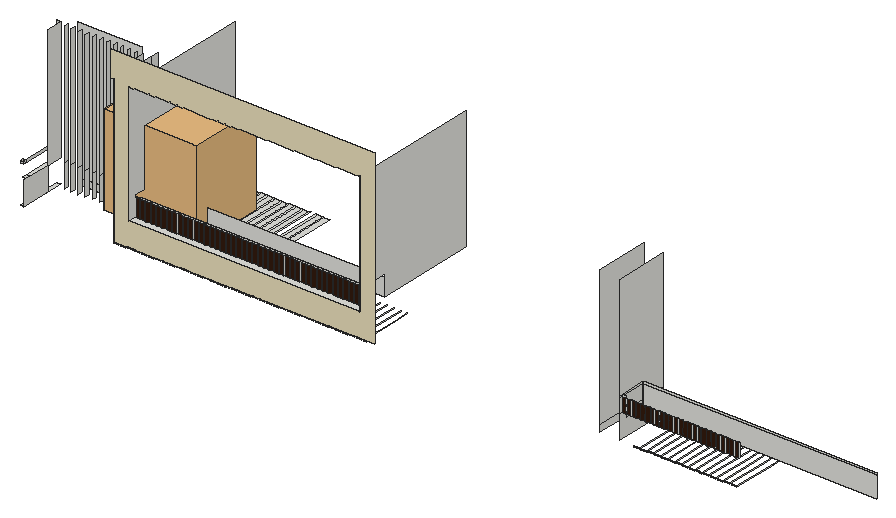
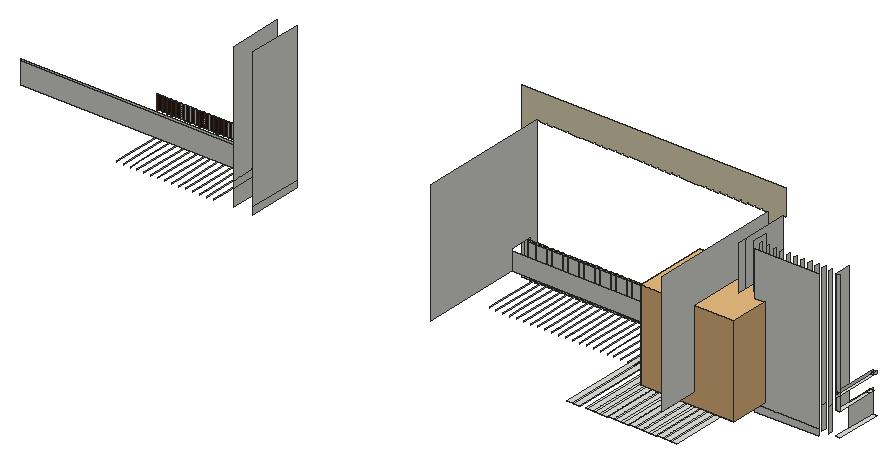
# SketchUp Ruby script. Lengths in inches.
U = 1.inch
M = Sketchup.active_model
def pt(a) = Geom::Point3d.new(a.map { |v| v * U })
def face(e, loops, mat)
  f = e.add_face(loops[0].map { |a| pt(a) })
  loops[1..].each { |l| e.add_face(l.map { |a| pt(a) }).erase! }
  f.material = f.back_material = mat if mat
  f
end
# faces: each face lists its corners as indices into pts; further lists are holes
def faces(e, pts, list, mat = nil) = list.each { |f| face(e, (f[0].is_a?(Array) ? f : [f]).map { |l| l.map { |i| pts[i] } }, mat) }
# xy, xz, yz: faces in a plane at the given z, y or x. An outline is a flat list of corners, or four numbers for a rectangle; further outlines are holes
def ring(l) = l.size == 4 ? [[l[0], l[1]], [l[2], l[1]], [l[2], l[3]], [l[0], l[3]]] : l.each_slice(2).to_a
def flat(e, list, mat, &to3) = list.each { |f| face(e, (f[0].is_a?(Array) ? f : [f]).map { |l| ring(l).map { |u, v| to3.(u, v) } }, mat) }
def xy(e, z, list, mat = nil) = flat(e, list, mat) { |x, y| [x, y, z] }
def xz(e, y, list, mat = nil) = flat(e, list, mat) { |x, z| [x, y, z] }
def yz(e, x, list, mat = nil) = flat(e, list, mat) { |y, z| [x, y, z] }
def lines(e, pts, list) = list.each { |a, b| e.add_line(pt(pts[a]), pt(pts[b])) }
# prism: a flat outline (further loops are holes) pulled along v
def prism(e, loops, v, mat = nil)
  f = face(e, loops, mat); d = Geom::Vector3d.new(v.map { |x| x * U })
  f.pushpull(f.normal.samedirection?(d) ? d.length : -d.length)
end
def box(e, o, s, mat = nil) = prism(e, [[o, [o[0] + s[0], o[1], o[2]], [o[0] + s[0], o[1] + s[1], o[2]], [o[0], o[1] + s[1], o[2]]]], [0, 0, s[2]], mat)
def at(x, y, z, deg = 0) = Geom::Transformation.translation(pt([x, y, z])) * Geom::Transformation.rotation(ORIGIN, Z_AXIS, deg.degrees)
def axes(o, x, y, z) = Geom::Transformation.new([*x, 0, *y, 0, *z, 0, *pt(o).to_a, 1])
def part(name) = M.definitions.add(name)
# library, detail: a bought-in or finely detailed component or shape, given as its bounding box
def library(name, o, s) = part(name).tap { |d| box(d.entities, o, s) }
def detail(e, o, s) = box(e.add_group.entities, o, s)
def put(e, d, t, mat = nil) = e.add_instance(d, t).tap { |i| i.material = mat if mat }
def group(e, t, mat = nil) = e.add_group.tap { |g| g.transformation = t; g.material = mat if mat }.entities
root = M.entities
M.materials.add("[Color D01]").color = [237, 225, 189]
M.materials.add("[Wood Veneer 01]").color = [51, 28, 15]
c1 = library("Round Planter with Plant",[-35.48,-39.77,0],[80.62,63.55,77.875])
xy(root,254.6875,[[1049,246.64,1052.37,286.21],[1130.14,246.64,1134.52,361.27],[1134.52,246.64,1136.14,361.27],[1136.14,246.64,1140.52,361.27],[1140.52,246.64,1142.14,361.27],
  [1142.14,246.64,1146.52,361.27],[1146.52,246.64,1148.14,361.27],[1148.14,246.64,1152.52,361.27],[1152.52,246.64,1154.14,361.27],[1154.14,246.64,1158.52,361.27],
  [1158.52,246.64,1160.14,361.27],[1160.14,246.64,1164.52,361.27],[1164.52,246.64,1166.14,361.27],[1166.14,246.64,1170.52,361.27],[1170.52,246.64,1172.14,361.27],
  [1172.14,246.64,1176.52,361.27],[1176.52,246.64,1178.14,361.27],[1178.14,246.64,1182.52,361.27],[1182.52,246.64,1184.14,361.27],[1184.14,246.64,1188.52,361.27],
  [1188.52,246.64,1190.14,361.27],[1190.14,246.64,1194.52,361.27],[1194.52,246.64,1196.14,361.27],[1196.14,246.64,1200.52,361.27],[1200.52,246.64,1202.14,361.27],
  [1202.14,246.64,1206.52,361.27],[1206.52,246.64,1208.14,361.27],[1212.52,246.64,1214.14,361.27],[1214.14,246.64,1218.52,361.27],[1218.52,246.64,1220.14,361.27],
  [1220.14,246.64,1224.52,361.27]])
xy(root,275.125,[[1142.89,246.64,1342.64,246.64,1342.64,255.84,1146.57,255.84,1146.57,253.84,1142.89,253.84],[1049,249.27,1052.37,253.58],[1049,253.58,1052.37,286.21],[1142.89,253.84,1146.57,255.47]])
xy(root,287.25,[[1049,246.64,1051.625,249.27],[1049,249.27,1051.625,286.21]])
xz(root,246.64,[[1049,287.25,1051.625,289.1875]])
xz(root,246.64,[[[1130.14,254.6875,1355.5625,254.6875,1355.5625,403.1875,1127.51,403.1875,1127.51,380.6875,1130.14,380.6875],[1142.89,275.125,1142.89,379.5625,1147.3,379.5625,1147.3,380.6875,1148.89,380.6875,1148.89,379.5625,1153.3,379.5625,1153.3,380.6875,1154.89,380.6875,1154.89,379.5625,1159.3,379.5625,1159.3,380.6875,1160.89,380.6875,1160.89,379.5625,1165.3,379.5625,1165.3,380.6875,1166.89,380.6875,1166.89,379.5625,1171.3,379.5625,1171.3,380.6875,1172.89,380.6875,1172.89,379.5625,1177.3,379.5625,1177.3,380.6875,1178.89,380.6875,1178.89,379.5625,1183.3,379.5625,1183.3,380.6875,1184.89,380.6875,1184.89,379.5625,1189.3,379.5625,1189.3,380.6875,1190.89,380.6875,1190.89,379.5625,1195.3,379.5625,1195.3,380.6875,1196.89,380.6875,1196.89,379.5625,1201.3,379.5625,1201.3,380.6875,1202.89,380.6875,1202.89,379.5625,1207.3,379.5625,1207.3,380.6875,1208.89,380.6875,1208.89,379.5625,1213.3,379.5625,1213.3,380.6875,1214.89,380.6875,1214.89,379.5625,1219.3,379.5625,1219.3,380.6875,1220.89,380.6875,1220.89,379.5625,1225.3,379.5625,1225.3,380.6875,1226.89,380.6875,1226.89,379.5625,1231.3,379.5625,1231.3,380.6875,1232.89,380.6875,1232.89,379.5625,1237.3,379.5625,1237.3,380.6875,1238.89,380.6875,1238.89,380.0625,1243.3,380.0625,1243.3,380.6875,1244.89,380.6875,1244.89,380.0625,1249.3,380.0625,1249.3,380.6875,1250.89,380.6875,1250.89,380.0625,1255.3,380.0625,1255.3,380.6875,1256.89,380.6875,1256.89,380.0625,1261.3,380.0625,1261.3,380.6875,1262.89,380.6875,1262.89,380.0625,1267.3,380.0625,1267.3,380.6875,1268.89,380.6875,1268.89,380.0625,1273.3,380.0625,1273.3,380.6875,1274.89,380.6875,1274.89,380.0625,1279.3,380.0625,1279.3,380.6875,1280.89,380.6875,1280.89,380.0625,1285.3,380.0625,1285.3,380.6875,1286.89,380.6875,1286.89,380.0625,1291.3,380.0625,1291.3,380.6875,1292.89,380.6875,1292.89,380.0625,1297.3,380.0625,1297.3,380.6875,1298.89,380.6875,1298.89,380.0625,1303.3,380.0625,1303.3,380.6875,1304.89,380.6875,1304.89,380.1875,1309.3,380.1875,1309.3,380.6875,1310.89,380.6875,1310.89,380.1875,1315.3,380.1875,1315.3,380.6875,1316.89,380.6875,1316.89,380.1875,1321.3,380.1875,1321.3,380.6875,1322.89,380.6875,1322.89,380.1875,1327.3,380.1875,1327.3,380.6875,1328.89,380.6875,1328.89,380.1875,1333.3,380.1875,1333.3,380.6875,1334.89,380.6875,1334.89,380.1875,1339.3,380.1875,1339.3,380.6875,1342.64,380.6875,1342.64,275.125]]],"[Color D01]")
xz(root,246.64,[[1130.14,253.9375,1134.52,254.6875],[1136.14,253.9375,1140.52,254.6875],[1142.14,253.9375,1146.52,254.6875],[1148.14,253.9375,1152.52,254.6875],[1154.14,253.9375,1158.52,254.6875],
  [1160.14,253.9375,1164.52,254.6875],[1166.14,253.9375,1170.52,254.6875],[1172.14,253.9375,1176.52,254.6875],[1178.14,253.9375,1182.52,254.6875],[1184.14,253.9375,1188.52,254.6875],
  [1190.14,253.9375,1194.52,254.6875],[1196.14,253.9375,1200.52,254.6875],[1202.14,253.9375,1206.52,254.6875],[1208.14,253.9375,1212.52,254.6875],[1214.14,253.9375,1218.52,254.6875],
  [1220.14,253.9375,1224.52,254.6875],[1226.14,253.9375,1230.52,254.6875],[1232.14,253.9375,1236.52,254.6875],[1238.14,253.9375,1242.52,254.6875],[1244.14,253.9375,1248.52,254.6875],
  [1250.14,253.9375,1254.52,254.6875],[1256.14,253.9375,1260.52,254.6875],[1262.14,253.9375,1266.52,254.6875],[1268.14,253.9375,1272.52,254.6875],[1274.14,253.9375,1278.52,254.6875],
  [1280.14,253.9375,1284.52,254.6875],[1286.14,253.9375,1290.52,254.6875],[1292.14,253.9375,1296.52,254.6875],[1298.14,253.9375,1302.52,254.6875],[1304.14,253.9375,1308.52,254.6875],
  [1310.14,253.9375,1314.52,254.6875],[1316.14,253.9375,1320.52,254.6875],[1322.14,253.9375,1326.52,254.6875],[1328.14,253.9375,1332.52,254.6875],[1334.14,253.9375,1338.52,254.6875],
  [1340.14,253.9375,1344.52,254.6875],[1346.14,253.9375,1348.32,254.6875],[1579.81,253.9375,1584.56,254.6875],[1585.81,253.9375,1590.56,254.6875],[1591.81,253.9375,1596.56,254.6875],
  [1597.81,253.9375,1602.56,254.6875],[1603.81,253.9375,1608.56,254.6875],[1609.81,253.9375,1614.56,254.6875],[1615.81,253.9375,1620.56,254.6875],[1621.81,253.9375,1626.56,254.6875],
  [1627.81,253.9375,1632.56,254.6875],[1633.81,253.9375,1638.56,254.6875],[1639.81,253.9375,1644.56,254.6875],[1645.81,253.9375,1650.56,254.6875],[1651.81,253.9375,1656.56,254.6875],
  [1657.81,253.9375,1662.56,254.6875],[1663.81,253.9375,1668.56,254.6875]],"[Wood Veneer 01]")
xz(root,249.27,[[1570.58,275.125,1571.36,287.25],[1574.64,275.125,1575.43,287.25],[1578.7,275.125,1579.49,287.25],[1582.77,275.125,1583.55,287.25],[1586.83,275.125,1587.61,287.25],
  [1590.89,275.125,1591.68,287.25],[1594.95,275.125,1595.74,287.25],[1599.02,275.125,1599.8,287.25],[1603.08,275.125,1603.86,287.25],[1607.14,275.125,1607.93,287.25],
  [1611.2,275.125,1611.99,287.25],[1615.27,275.125,1616.05,287.25],[1619.33,275.125,1620.11,287.25],[1623.39,275.125,1624.18,287.25],[1627.45,275.125,1628.24,287.25],
  [1631.52,275.125,1632.3,287.25],[1635.58,275.125,1636.36,287.25],[1639.64,275.125,1640.43,287.25],[1643.7,275.125,1644.49,287.25],[1647.77,275.125,1648.55,287.25],
  [1651.83,275.125,1652.61,287.25],[1655.89,275.125,1656.68,287.25],[1659.95,275.125,1660.74,287.25],[1664.02,275.125,1664.8,287.25],[1668.08,275.125,1668.86,287.25],
  [1049,287.25,1051.625,289.1875],[1567.3,287.25,1570.58,289.1875]])
xz(root,249.27,[[1567.3,275.125,1570.58,287.25],[1571.36,275.125,1574.64,287.25],[1575.43,275.125,1578.7,287.25],[1579.49,275.125,1582.77,287.25],[1583.55,275.125,1586.83,287.25],
  [1587.61,275.125,1590.89,287.25],[1591.68,275.125,1594.95,287.25],[1595.74,275.125,1599.02,287.25],[1599.8,275.125,1603.08,287.25],[1603.86,275.125,1607.14,287.25],
  [1607.93,275.125,1611.2,287.25],[1611.99,275.125,1615.27,287.25],[1616.05,275.125,1619.33,287.25],[1620.11,275.125,1623.39,287.25],[1624.18,275.125,1627.45,287.25],
  [1628.24,275.125,1631.52,287.25],[1632.3,275.125,1635.58,287.25],[1636.36,275.125,1639.64,287.25],[1640.43,275.125,1643.7,287.25],[1644.49,275.125,1647.77,287.25],
  [1648.55,275.125,1651.83,287.25],[1652.61,275.125,1655.89,287.25],[1656.68,275.125,1659.95,287.25],[1660.74,275.125,1664.02,287.25],[1664.8,275.125,1668.08,287.25]],"[Wood Veneer 01]")
xz(root,253.84,[[1142.89,275.125,1146.57,290.375],[1147.51,275.125,1151.2,290.375],[1152.14,275.125,1155.82,290.375],[1156.76,275.125,1160.45,290.375],[1161.39,275.125,1165.07,290.375],
  [1166.01,275.125,1169.7,290.375],[1170.64,275.125,1174.32,290.375],[1175.26,275.125,1178.95,290.375],[1179.89,275.125,1183.57,290.375],[1184.51,275.125,1188.2,290.375],
  [1189.14,275.125,1192.82,290.375],[1193.76,275.125,1197.45,290.375],[1198.39,275.125,1202.07,290.375],[1203.01,275.125,1206.7,290.375],[1207.64,275.125,1211.32,290.375],
  [1212.26,275.125,1215.95,290.375],[1216.89,275.125,1220.57,290.375],[1221.51,275.125,1225.2,290.375],[1226.14,275.125,1229.82,290.375],[1230.76,275.125,1234.45,290.375],
  [1235.39,275.125,1239.07,290.375],[1240.01,275.125,1243.7,290.375],[1244.64,275.125,1248.32,290.375],[1249.26,275.125,1252.95,290.375],[1253.89,275.125,1257.57,290.375],
  [1258.51,275.125,1262.2,290.375],[1263.14,275.125,1266.82,290.375],[1267.76,275.125,1271.45,290.375],[1272.39,275.125,1276.07,290.375],[1277.01,275.125,1280.7,290.375],
  [1281.64,275.125,1285.32,290.375],[1286.26,275.125,1289.95,290.375],[1290.89,275.125,1294.57,290.375],[1295.51,275.125,1299.2,290.375],[1300.14,275.125,1303.82,290.375],
  [1304.76,275.125,1308.45,290.375],[1309.39,275.125,1313.07,290.375],[1314.01,275.125,1317.7,290.375],[1318.64,275.125,1322.32,290.375],[1323.26,275.125,1326.95,290.375],
  [1327.89,275.125,1331.57,290.375],[1332.51,275.125,1336.2,290.375],[1337.14,275.125,1340.82,290.375],[1341.76,275.125,1345.45,290.375]],"[Wood Veneer 01]")
xz(root,255.47,[[1142.89,275.125,1146.57,290.375]])
xz(root,255.84,[[1146.57,275.125,1342.64,290.375]])
xz(root,271.8,[[1567.3,269.0625,1769.03,287.25],[1567.3,287.25,1769.03,289.1875]])
xz(root,273.33,[[1142.89,275.125,1342.64,290.375]])
xz(root,286.21,[[1049,275.125,1052.37,275.125,1052.37,380.6875,1049,380.6875,1049,289.1875,1051.625,289.1875,1051.625,287.25,1049,287.25],[1049,287.25,1051.625,289.1875]])
xz(root,293.45,[[1061.59,254.6875,1116.3,260.6875],[1061.59,260.6875,1116.3,380.6875]])
yz(root,1049,[[246.64,287.25,249.27,289.1875],[286.21,287.25,290.02,289.1875]])
yz(root,1051.625,[[246.64,287.25,249.27,289.1875],[249.27,287.25,286.21,289.1875]])
yz(root,1052.37,[[246.64,254.6875,271.96,275.125],[271.96,275.125,286.21,380.6875]])
yz(root,1058.37,[[282.52,254.6875,286.21,275.125],[282.52,275.125,286.21,380.6875]])
yz(root,1064.37,[[282.52,254.6875,286.21,275.125],[282.52,275.125,286.21,380.6875]])
yz(root,1070.37,[[282.52,254.6875,286.21,275.125],[282.52,275.125,286.21,380.6875]])
yz(root,1076.37,[[282.52,254.6875,286.21,275.125],[282.52,275.125,286.21,380.6875]])
yz(root,1082.37,[[283.46,254.6875,286.21,275.125],[283.46,275.125,286.21,380.6875]])
yz(root,1088.37,[[283.46,254.6875,286.21,275.125],[283.46,275.125,286.21,380.6875]])
yz(root,1094.37,[[283.46,254.6875,286.21,275.125],[283.46,275.125,286.21,380.6875]])
yz(root,1100.37,[[283.46,254.6875,286.21,275.125],[283.46,275.125,286.21,380.6875]])
yz(root,1106.37,[[283.46,254.6875,286.21,275.125],[283.46,275.125,286.21,380.6875]])
yz(root,1112.37,[[283.46,254.6875,286.21,275.125],[283.46,275.125,286.21,380.6875]])
yz(root,1118.37,[[283.46,254.6875,286.21,275.125],[283.46,275.125,286.21,380.6875]])
yz(root,1123.68,[[272.89,254.6875,286.21,275.125],[272.89,275.125,286.21,380.6875]])
yz(root,1130.14,[[246.64,253.9375,286.21,254.6875],[286.21,253.9375,293.45,254.6875],[246.64,254.6875,286.21,260.6875],[286.21,254.6875,293.45,260.6875],[246.64,260.6875,286.21,380.6875],
  [286.21,260.6875,293.45,380.6875]])
yz(root,1136.14,[[246.64,253.9375,286.21,254.6875],[286.21,253.9375,293.45,254.6875]])
yz(root,1142.14,[[246.64,253.9375,286.21,254.6875],[286.21,253.9375,293.45,254.6875]])
yz(root,1142.89,[[246.64,275.125,253.84,275.125,253.84,290.375,253.22,290.375,253.22,292.5625,273.33,292.5625,273.33,275.125,361.27,275.125,361.27,379.5625,246.64,379.5625],[253.84,275.125,255.47,290.375]])
yz(root,1146.57,[[253.84,275.125,255.47,290.375],[255.47,275.125,255.84,290.375]])
yz(root,1148.14,[[246.64,253.9375,286.21,254.6875],[286.21,253.9375,293.45,254.6875]])
yz(root,1151.2,[[253.84,275.125,255.47,290.375]])
yz(root,1154.14,[[246.64,253.9375,286.21,254.6875],[286.21,253.9375,293.45,254.6875]])
yz(root,1155.82,[[253.84,275.125,255.47,290.375]])
yz(root,1160.14,[[246.64,253.9375,286.21,254.6875],[286.21,253.9375,293.45,254.6875]])
yz(root,1160.45,[[253.84,275.125,255.47,290.375]])
yz(root,1165.07,[[253.84,275.125,255.47,290.375]])
yz(root,1166.14,[[246.64,253.9375,286.21,254.6875],[286.21,253.9375,293.45,254.6875]])
yz(root,1169.7,[[253.84,275.125,255.47,290.375]])
yz(root,1172.14,[[246.64,253.9375,286.21,254.6875],[286.21,253.9375,293.45,254.6875]])
yz(root,1174.32,[[253.84,275.125,255.47,290.375]])
yz(root,1178.14,[[246.64,253.9375,286.21,254.6875],[286.21,253.9375,293.45,254.6875]])
yz(root,1178.95,[[253.84,275.125,255.47,290.375]])
yz(root,1183.57,[[253.84,275.125,255.47,290.375]])
yz(root,1184.14,[[246.64,253.9375,286.21,254.6875],[286.21,253.9375,293.45,254.6875]])
yz(root,1188.2,[[253.84,275.125,255.47,290.375]])
yz(root,1190.14,[[246.64,253.9375,286.21,254.6875],[286.21,253.9375,293.45,254.6875]])
yz(root,1192.82,[[253.84,275.125,255.47,290.375]])
yz(root,1196.14,[[246.64,253.9375,286.21,254.6875],[286.21,253.9375,293.45,254.6875]])
yz(root,1197.45,[[253.84,275.125,255.47,290.375]])
yz(root,1202.07,[[253.84,275.125,255.47,290.375]])
yz(root,1202.14,[[246.64,253.9375,286.21,254.6875],[286.21,253.9375,293.45,254.6875]])
yz(root,1206.7,[[253.84,275.125,255.47,290.375]])
yz(root,1208.14,[[246.64,253.9375,286.21,254.6875],[286.21,253.9375,293.45,254.6875]])
yz(root,1211.32,[[253.84,275.125,255.47,290.375]])
yz(root,1214.14,[[246.64,253.9375,286.21,254.6875],[286.21,253.9375,293.45,254.6875]])
yz(root,1215.95,[[253.84,275.125,255.47,290.375]])
yz(root,1220.14,[[246.64,253.9375,286.21,254.6875],[286.21,253.9375,293.45,254.6875]])
yz(root,1220.57,[[253.84,275.125,255.47,290.375]])
yz(root,1225.2,[[253.84,275.125,255.47,290.375]])
yz(root,1226.14,[[246.64,253.9375,286.21,254.6875],[286.21,253.9375,293.45,254.6875]])
yz(root,1229.82,[[253.84,275.125,255.47,290.375]])
yz(root,1232.14,[[246.64,253.9375,286.21,254.6875],[286.21,253.9375,293.45,254.6875]])
yz(root,1234.45,[[253.84,275.125,255.47,290.375]])
yz(root,1238.14,[[246.64,253.9375,286.21,254.6875],[286.21,253.9375,293.45,254.6875]])
yz(root,1239.07,[[253.84,275.125,255.47,290.375]])
yz(root,1243.7,[[253.84,275.125,255.47,290.375]])
yz(root,1244.14,[[246.64,253.9375,286.21,254.6875],[286.21,253.9375,293.45,254.6875]])
yz(root,1248.32,[[253.84,275.125,255.47,290.375]])
yz(root,1250.14,[[246.64,253.9375,286.21,254.6875],[286.21,253.9375,293.45,254.6875]])
yz(root,1252.95,[[253.84,275.125,255.47,290.375]])
yz(root,1256.14,[[246.64,253.9375,286.21,254.6875],[286.21,253.9375,293.45,254.6875]])
yz(root,1257.57,[[253.84,275.125,255.47,290.375]])
yz(root,1262.14,[[246.64,253.9375,286.21,254.6875],[286.21,253.9375,293.45,254.6875]])
yz(root,1262.2,[[253.84,275.125,255.47,290.375]])
yz(root,1266.82,[[253.84,275.125,255.47,290.375]])
yz(root,1268.14,[[246.64,253.9375,286.21,254.6875],[286.21,253.9375,293.45,254.6875]])
yz(root,1271.45,[[253.84,275.125,255.47,290.375]])
yz(root,1274.14,[[246.64,253.9375,286.21,254.6875],[286.21,253.9375,293.45,254.6875]])
yz(root,1276.07,[[253.84,275.125,255.47,290.375]])
yz(root,1280.14,[[246.64,253.9375,286.21,254.6875],[286.21,253.9375,293.45,254.6875]])
yz(root,1280.7,[[253.84,275.125,255.47,290.375]])
yz(root,1285.32,[[253.84,275.125,255.47,290.375]])
yz(root,1286.14,[[246.64,253.9375,286.21,254.6875],[286.21,253.9375,293.45,254.6875]])
yz(root,1289.95,[[253.84,275.125,255.47,290.375]])
yz(root,1292.14,[[246.64,253.9375,286.21,254.6875],[286.21,253.9375,293.45,254.6875]])
yz(root,1294.57,[[253.84,275.125,255.47,290.375]])
yz(root,1298.14,[[246.64,253.9375,286.21,254.6875],[286.21,253.9375,293.45,254.6875]])
yz(root,1299.2,[[253.84,275.125,255.47,290.375]])
yz(root,1303.82,[[253.84,275.125,255.47,290.375]])
yz(root,1304.14,[[246.64,253.9375,286.21,254.6875],[286.21,253.9375,293.45,254.6875]])
yz(root,1308.45,[[253.84,275.125,255.47,290.375]])
yz(root,1310.14,[[246.64,253.9375,286.21,254.6875],[286.21,253.9375,293.45,254.6875]])
yz(root,1313.07,[[253.84,275.125,255.47,290.375]])
yz(root,1316.14,[[246.64,253.9375,286.21,254.6875],[286.21,253.9375,293.45,254.6875]])
yz(root,1317.7,[[253.84,275.125,255.47,290.375]])
yz(root,1322.14,[[246.64,253.9375,286.21,254.6875],[286.21,253.9375,293.45,254.6875]])
yz(root,1322.32,[[253.84,275.125,255.47,290.375]])
yz(root,1326.95,[[253.84,275.125,255.47,290.375]])
yz(root,1328.14,[[246.64,253.9375,286.21,254.6875],[286.21,253.9375,293.45,254.6875]])
yz(root,1331.57,[[253.84,275.125,255.47,290.375]])
yz(root,1334.14,[[246.64,253.9375,286.21,254.6875],[286.21,253.9375,293.45,254.6875]])
yz(root,1336.2,[[253.84,275.125,255.47,290.375]])
yz(root,1340.14,[[246.64,253.9375,286.21,254.6875],[286.21,253.9375,293.45,254.6875]])
yz(root,1340.82,[[253.84,275.125,255.47,290.375]])
yz(root,1342.64,[[246.64,275.125,246.64,380.6875,361.27,380.6875,361.27,275.125,273.33,275.125,273.33,292.5625,253.22,292.5625,253.22,290.375,255.84,290.375,255.84,275.125]])
yz(root,1345.45,[[253.84,275.125,255.47,290.375]])
yz(root,1346.14,[[246.64,253.9375,286.21,254.6875],[286.21,253.9375,293.45,254.6875]])
yz(root,1550.25,[[246.64,254.6875,293.46,260.6875],[246.64,260.6875,293.46,380.6875]])
yz(root,1567.3,[[246.64,254.6875,293.46,254.6875,293.46,269.0625,253.58,269.0625,253.58,275.125,246.64,275.125],[253.58,269.0625,271.8,275.125],[271.8,269.0625,293.46,275.125],[246.64,275.125,249.27,287.25],[271.8,275.125,293.46,275.125,293.46,378.875,246.64,378.875,246.64,289.1875,271.8,289.1875],
  [249.27,275.125,271.8,287.25],[246.64,287.25,249.27,289.1875],[249.27,287.25,271.8,289.1875]])
yz(root,1584.56,[[246.64,253.9375,286.21,254.6875],[286.21,253.9375,293.45,254.6875]])
yz(root,1590.56,[[246.64,253.9375,286.21,254.6875],[286.21,253.9375,293.45,254.6875]])
yz(root,1596.56,[[246.64,253.9375,286.21,254.6875],[286.21,253.9375,293.45,254.6875]])
yz(root,1602.56,[[246.64,253.9375,286.21,254.6875],[286.21,253.9375,293.45,254.6875]])
yz(root,1608.56,[[246.64,253.9375,286.21,254.6875],[286.21,253.9375,293.45,254.6875]])
yz(root,1614.56,[[246.64,253.9375,286.21,254.6875],[286.21,253.9375,293.45,254.6875]])
yz(root,1620.56,[[246.64,253.9375,286.21,254.6875],[286.21,253.9375,293.45,254.6875]])
yz(root,1626.56,[[246.64,253.9375,286.21,254.6875],[286.21,253.9375,293.45,254.6875]])
yz(root,1632.56,[[246.64,253.9375,286.21,254.6875],[286.21,253.9375,293.45,254.6875]])
yz(root,1638.56,[[246.64,253.9375,286.21,254.6875],[286.21,253.9375,293.45,254.6875]])
yz(root,1644.56,[[246.64,253.9375,286.21,254.6875],[286.21,253.9375,293.45,254.6875]])
yz(root,1650.56,[[246.64,253.9375,286.21,254.6875],[286.21,253.9375,293.45,254.6875]])
yz(root,1656.56,[[246.64,253.9375,286.21,254.6875],[286.21,253.9375,293.45,254.6875]])
yz(root,1662.56,[[246.64,253.9375,286.21,254.6875],[286.21,253.9375,293.45,254.6875]])
yz(root,1668.56,[[246.64,253.9375,286.21,254.6875],[286.21,253.9375,293.45,254.6875]])
put(root,c1,at(1143.37,303,264.4375))
